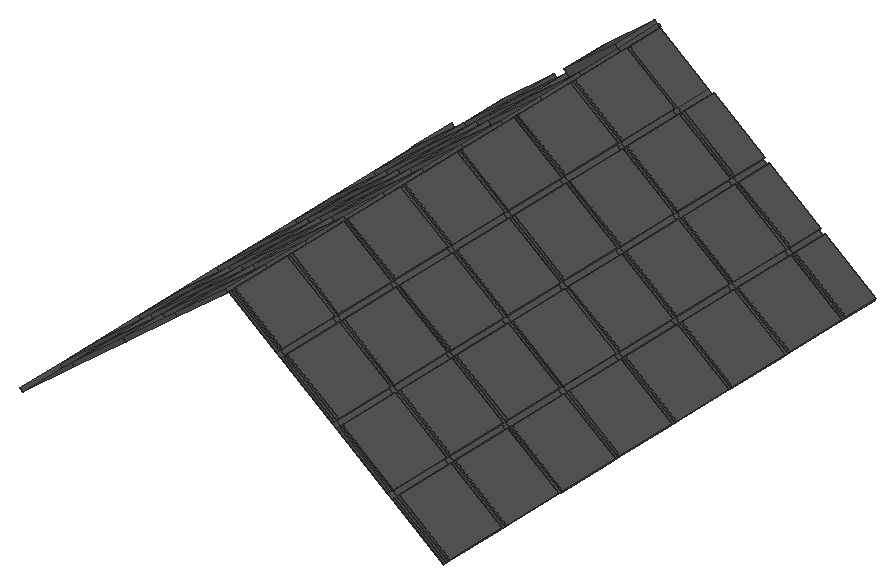
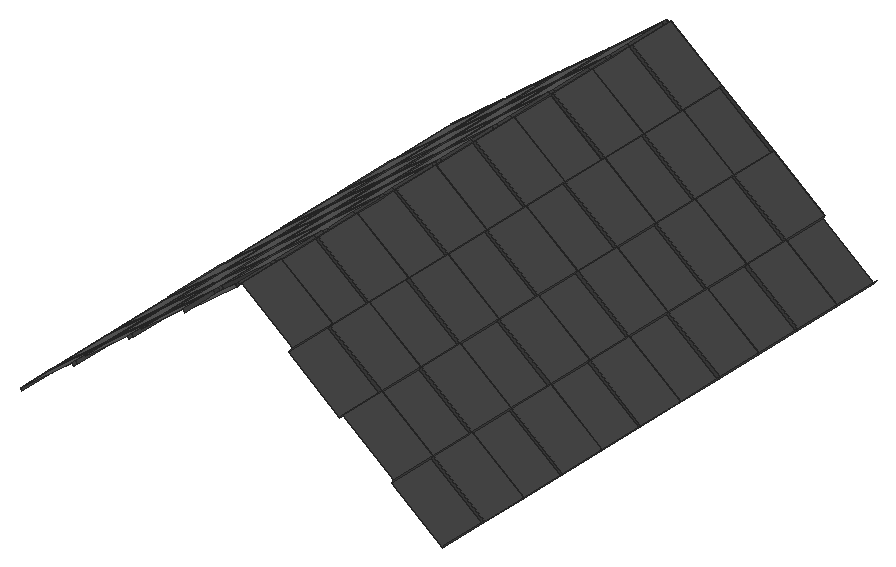
# SketchUp Ruby script. Lengths in inches.
U = 1.inch
M = Sketchup.active_model
def pt(a) = Geom::Point3d.new(a.map { |v| v * U })
def face(e, loops, mat)
  f = e.add_face(loops[0].map { |a| pt(a) })
  loops[1..].each { |l| e.add_face(l.map { |a| pt(a) }).erase! }
  f.material = f.back_material = mat if mat
  f
end
# faces: each face lists its corners as indices into pts; further lists are holes
def faces(e, pts, list, mat = nil) = list.each { |f| face(e, (f[0].is_a?(Array) ? f : [f]).map { |l| l.map { |i| pts[i] } }, mat) }
# xy, xz, yz: faces in a plane at the given z, y or x. An outline is a flat list of corners, or four numbers for a rectangle; further outlines are holes
def ring(l) = l.size == 4 ? [[l[0], l[1]], [l[2], l[1]], [l[2], l[3]], [l[0], l[3]]] : l.each_slice(2).to_a
def flat(e, list, mat, &to3) = list.each { |f| face(e, (f[0].is_a?(Array) ? f : [f]).map { |l| ring(l).map { |u, v| to3.(u, v) } }, mat) }
def xy(e, z, list, mat = nil) = flat(e, list, mat) { |x, y| [x, y, z] }
def xz(e, y, list, mat = nil) = flat(e, list, mat) { |x, z| [x, y, z] }
def yz(e, x, list, mat = nil) = flat(e, list, mat) { |y, z| [x, y, z] }
def lines(e, pts, list) = list.each { |a, b| e.add_line(pt(pts[a]), pt(pts[b])) }
# prism: a flat outline (further loops are holes) pulled along v
def prism(e, loops, v, mat = nil)
  f = face(e, loops, mat); d = Geom::Vector3d.new(v.map { |x| x * U })
  f.pushpull(f.normal.samedirection?(d) ? d.length : -d.length)
end
def box(e, o, s, mat = nil) = prism(e, [[o, [o[0] + s[0], o[1], o[2]], [o[0] + s[0], o[1] + s[1], o[2]], [o[0], o[1] + s[1], o[2]]]], [0, 0, s[2]], mat)
def at(x, y, z, deg = 0) = Geom::Transformation.translation(pt([x, y, z])) * Geom::Transformation.rotation(ORIGIN, Z_AXIS, deg.degrees)
def axes(o, x, y, z) = Geom::Transformation.new([*x, 0, *y, 0, *z, 0, *pt(o).to_a, 1])
def part(name) = M.definitions.add(name)
# library, detail: a bought-in or finely detailed component or shape, given as its bounding box
def library(name, o, s) = part(name).tap { |d| box(d.entities, o, s) }
def detail(e, o, s) = box(e.add_group.entities, o, s)
def put(e, d, t, mat = nil) = e.add_instance(d, t).tap { |i| i.material = mat if mat }
def group(e, t, mat = nil) = e.add_group.tap { |g| g.transformation = t; g.material = mat if mat }.entities
root = M.entities
M.materials.add("[Color M06]").color = [86, 86, 86]
xz(root,343.1875,[[320.63,393.75,339.53,408.54,339.04,409.17,338.73,409.57,319.83,394.78],[339.53,408.54,339.04,409.17,338.73,409.57,357.63,424.36,357.9375,423.97,358.43,423.34],[358.43,423.34,377.33,438.125,376.53,439.15,357.63,424.36,357.9375,423.97]],"[Color M06]")
xz(root,343.375,[[456.38,376.26,437.48,391.05,438.1,391.84,457,377.05],[435.9,392.29,417,407.08,417.62,407.87,436.52,393.07],[415.43,408.3125,396.53,423.1,397.15,423.89,416.05,409.1],[394.95,424.33,377.33,438.125,377.95,438.91,395.57,425.12]],"[Color M06]")
xz(root,345.375,[[456.38,376.26,457,377.05,438.1,391.84,437.48,391.05],[435.9,392.29,436.52,393.07,417.62,407.87,417,407.08],[415.43,408.3125,416.05,409.1,397.15,423.89,396.53,423.1],[394.95,424.33,395.57,425.12,377.95,438.91,377.33,438.125]],"[Color M06]")
xz(root,361.1875,[[301.73,378.96,320.63,393.75,320.14,394.38,319.83,394.78,300.93,379.98,301.24,379.59],[320.63,393.75,320.14,394.38,319.83,394.78,338.73,409.57,339.04,409.17,339.53,408.54],[339.53,408.54,358.43,423.34,357.9375,423.97,357.63,424.36,338.73,409.57,339.04,409.17],[358.43,423.34,357.9375,423.97,357.63,424.36,376.53,439.15,377.33,438.125]],"[Color M06]")
xz(root,369.375,[[456.38,376.26,437.48,391.05,438.1,391.84,457,377.05],[435.9,392.29,417,407.08,417.62,407.87,436.52,393.07],[415.43,408.3125,396.53,423.1,397.15,423.89,416.05,409.1],[394.95,424.33,377.33,438.125,377.95,438.91,395.57,425.12]],"[Color M06]")
xz(root,371.375,[[456.38,376.26,457,377.05,438.1,391.84,437.48,391.05],[435.9,392.29,436.52,393.07,417.62,407.87,417,407.08],[415.43,408.3125,416.05,409.1,397.15,423.89,396.53,423.1],[394.95,424.33,395.57,425.12,377.95,438.91,377.33,438.125]],"[Color M06]")
xz(root,379.1875,[[301.73,378.96,301.24,379.59,300.93,379.98,319.83,394.78,320.14,394.38,320.63,393.75],[320.63,393.75,339.53,408.54,339.04,409.17,338.73,409.57,319.83,394.78,320.14,394.38],[339.53,408.54,339.04,409.17,338.73,409.57,357.63,424.36,357.9375,423.97,358.43,423.34],[358.43,423.34,377.33,438.125,376.53,439.15,357.63,424.36,357.9375,423.97]],"[Color M06]")
xz(root,395.375,[[456.38,376.26,437.48,391.05,438.1,391.84,457,377.05],[435.9,392.29,417,407.08,417.62,407.87,436.52,393.07],[415.43,408.3125,396.53,423.1,397.15,423.89,416.05,409.1],[394.95,424.33,377.33,438.125,377.95,438.91,395.57,425.12]],"[Color M06]")
xz(root,397.1875,[[301.73,378.96,320.63,393.75,320.14,394.38,319.83,394.78,300.93,379.98,301.24,379.59],[320.63,393.75,320.14,394.38,319.83,394.78,338.73,409.57,339.04,409.17,339.53,408.54],[339.53,408.54,358.43,423.34,357.9375,423.97,357.63,424.36,338.73,409.57,339.04,409.17],[358.43,423.34,357.9375,423.97,357.63,424.36,376.53,439.15,377.33,438.125]],"[Color M06]")
xz(root,397.375,[[456.38,376.26,457,377.05,438.1,391.84,437.48,391.05],[435.9,392.29,436.52,393.07,417.62,407.87,417,407.08],[415.43,408.3125,416.05,409.1,397.15,423.89,396.53,423.1],[394.95,424.33,395.57,425.12,377.95,438.91,377.33,438.125]],"[Color M06]")
xz(root,415.1875,[[301.73,378.96,301.24,379.59,300.93,379.98,319.83,394.78,320.63,393.75],[320.63,393.75,339.53,408.54,338.73,409.57,319.83,394.78],[339.53,408.54,338.73,409.57,357.63,424.36,357.9375,423.97,358.43,423.34],[358.43,423.34,377.33,438.125,376.53,439.15,357.63,424.36,357.9375,423.97]],"[Color M06]")
xz(root,421.375,[[456.38,376.26,437.48,391.05,438.1,391.84,457,377.05],[435.9,392.29,417,407.08,417.62,407.87,436.52,393.07],[415.43,408.3125,396.53,423.1,397.15,423.89,416.05,409.1],[394.95,424.33,377.33,438.125,377.95,438.91,395.57,425.12]],"[Color M06]")
xz(root,423.375,[[456.38,376.26,457,377.05,438.1,391.84,437.48,391.05],[435.9,392.29,436.52,393.07,417.62,407.87,417,407.08],[415.43,408.3125,416.05,409.1,397.15,423.89,396.53,423.1],[394.95,424.33,395.57,425.12,377.95,438.91,377.33,438.125]],"[Color M06]")
xz(root,433.1875,[[301.73,378.96,320.63,393.75,319.83,394.78,300.93,379.98,301.24,379.59],[320.63,393.75,319.83,394.78,338.73,409.57,339.53,408.54],[339.53,408.54,358.43,423.34,357.9375,423.97,357.63,424.36,338.73,409.57],[358.43,423.34,357.9375,423.97,357.63,424.36,376.53,439.15,377.33,438.125]],"[Color M06]")
xz(root,447.375,[[456.38,376.26,437.48,391.05,438.1,391.84,457,377.05],[435.9,392.29,417,407.08,417.62,407.87,436.52,393.07],[415.43,408.3125,396.53,423.1,397.15,423.89,416.05,409.1],[394.95,424.33,377.33,438.125,377.95,438.91,395.57,425.12]],"[Color M06]")
xz(root,449.375,[[456.38,376.26,457,377.05,438.1,391.84,437.48,391.05],[435.9,392.29,436.52,393.07,417.62,407.87,417,407.08],[415.43,408.3125,416.05,409.1,397.15,423.89,396.53,423.1],[394.95,424.33,395.57,425.12,377.95,438.91,377.33,438.125]],"[Color M06]")
xz(root,451.1875,[[301.73,378.96,301.24,379.59,300.93,379.98,319.83,394.78,320.14,394.38,320.63,393.75],[320.63,393.75,339.53,408.54,339.04,409.17,338.73,409.57,319.83,394.78,320.14,394.38],[339.53,408.54,339.04,409.17,338.73,409.57,357.63,424.36,358.43,423.34],[358.43,423.34,377.33,438.125,376.53,439.15,357.63,424.36]],"[Color M06]")
xz(root,469.1875,[[301.73,378.96,320.63,393.75,320.14,394.38,319.83,394.78,300.93,379.98,301.24,379.59],[320.63,393.75,320.14,394.38,319.83,394.78,338.73,409.57,339.04,409.17,339.53,408.54],[339.53,408.54,358.43,423.34,357.63,424.36,338.73,409.57,339.04,409.17],[358.43,423.34,357.63,424.36,376.53,439.15,377.33,438.125]],"[Color M06]")
xz(root,473.375,[[456.38,376.26,437.48,391.05,438.1,391.84,457,377.05],[435.9,392.29,417,407.08,417.62,407.87,436.52,393.07],[415.43,408.3125,396.53,423.1,397.15,423.89,416.05,409.1],[394.95,424.33,377.33,438.125,377.95,438.91,395.57,425.12]],"[Color M06]")
xz(root,475.375,[[456.38,376.26,457,377.05,438.1,391.84,437.48,391.05],[435.9,392.29,436.52,393.07,417.62,407.87,417,407.08],[415.43,408.3125,416.05,409.1,397.15,423.89,396.53,423.1],[394.95,424.33,395.57,425.12,377.95,438.91,377.33,438.125]],"[Color M06]")
xz(root,487.1875,[[301.73,378.96,301.24,379.59,300.93,379.98,319.83,394.78,320.14,394.38,320.63,393.75],[320.63,393.75,339.53,408.54,339.04,409.17,338.73,409.57,319.83,394.78,320.14,394.38],[339.53,408.54,339.04,409.17,338.73,409.57,357.63,424.36,358.43,423.34],[358.43,423.34,377.33,438.125,376.53,439.15,357.63,424.36]],"[Color M06]")
xz(root,499.375,[[456.38,376.26,437.48,391.05,438.1,391.84,457,377.05],[435.9,392.29,417,407.08,417.62,407.87,436.52,393.07],[415.43,408.3125,396.53,423.1,397.15,423.89,416.05,409.1],[394.95,424.33,377.33,438.125,377.95,438.91,395.57,425.12]],"[Color M06]")
xz(root,501.375,[[456.38,376.26,457,377.05,438.1,391.84,437.48,391.05],[435.9,392.29,436.52,393.07,417.62,407.87,417,407.08],[415.43,408.3125,416.05,409.1,397.15,423.89,396.53,423.1],[394.95,424.33,395.57,425.12,377.95,438.91,377.33,438.125]],"[Color M06]")
xz(root,505.1875,[[301.73,378.96,320.63,393.75,320.14,394.38,319.83,394.78,300.93,379.98,301.24,379.59],[320.63,393.75,320.14,394.38,319.83,394.78,338.73,409.57,339.04,409.17,339.53,408.54],[339.53,408.54,358.43,423.34,357.63,424.36,338.73,409.57,339.04,409.17],[358.43,423.34,357.63,424.36,376.53,439.15,377.33,438.125]],"[Color M06]")
xz(root,523.1875,[[301.73,378.96,301.24,379.59,300.93,379.98,319.83,394.78,320.14,394.38,320.63,393.75],[320.63,393.75,339.53,408.54,339.04,409.17,338.73,409.57,338.68,409.625,319.78,394.84,319.83,394.78,320.14,394.38],[339.53,408.54,339.04,409.17,338.73,409.57,357.63,424.36,357.9375,423.97,358.43,423.34],[358.43,423.34,377.33,438.125,376.53,439.15,375.68,440.23,356.78,425.44,357.63,424.36,357.9375,423.97]],"[Color M06]")
xz(root,525.375,[[456.38,376.26,437.48,391.05,438.1,391.84,457,377.05],[435.9,392.29,417,407.08,417.62,407.87,436.52,393.07],[415.43,408.3125,396.53,423.1,397.15,423.89,416.05,409.1],[394.95,424.33,377.33,438.125,377.95,438.91,395.57,425.12]],"[Color M06]")
xz(root,527.375,[[456.38,376.26,457,377.05,438.1,391.84,437.48,391.05],[435.9,392.29,436.52,393.07,417.62,407.87,417,407.08],[415.43,408.3125,416.05,409.1,397.15,423.89,396.53,423.1]],"[Color M06]")
xz(root,541.1875,[[377.33,438.125,377.95,438.91,377.09,439.59,376.53,439.15]],"[Color M06]")
p = [[456.38,345.375,376.26],[437.48,345.375,391.05],[437.48,343.375,391.05],[456.38,343.375,376.26],[456.38,369.375,376.26],[457,369.375,377.05],
  [457,345.375,377.05],[456.38,371.375,376.26],[437.48,371.375,391.05],[437.48,369.375,391.05],[456.38,395.375,376.26],[457,395.375,377.05],
  [457,371.375,377.05],[456.38,397.375,376.26],[437.48,397.375,391.05],[437.48,395.375,391.05],[456.38,421.375,376.26],[457,421.375,377.05],
  [457,397.375,377.05],[456.38,423.375,376.26],[437.48,423.375,391.05],[437.48,421.375,391.05],[456.38,447.375,376.26],[457,447.375,377.05],
  [457,423.375,377.05],[456.38,449.375,376.26],[437.48,449.375,391.05],[437.48,447.375,391.05],[456.38,473.375,376.26],[457,473.375,377.05],
  [457,449.375,377.05],[456.38,475.375,376.26],[437.48,475.375,391.05],[437.48,473.375,391.05],[456.38,499.375,376.26],[457,499.375,377.05],
  [457,475.375,377.05],[456.38,501.375,376.26],[437.48,501.375,391.05],[437.48,499.375,391.05],[456.38,525.375,376.26],[457,525.375,377.05],
  [457,501.375,377.05],[456.38,527.375,376.26],[437.48,527.375,391.05],[437.48,525.375,391.05],[456.38,541.1875,376.26],[457,541.1875,377.05],
  [457,527.375,377.05],[438.1,369.375,391.84],[438.1,345.375,391.84],[438.1,395.375,391.84],[438.1,371.375,391.84],[438.1,421.375,391.84],
  [438.1,397.375,391.84],[438.1,447.375,391.84],[438.1,423.375,391.84],[438.1,473.375,391.84],[438.1,449.375,391.84],[438.1,499.375,391.84],
  [438.1,475.375,391.84],[438.1,525.375,391.84],[438.1,501.375,391.84],[438.1,541.1875,391.84],[438.1,527.375,391.84],[301.73,343.1875,378.96],
  [301.73,361.1875,378.96],[301.24,361.1875,379.59],[300.93,361.1875,379.98],[300.93,343.1875,379.98],[320.63,361.1875,393.75],[320.63,343.1875,393.75],
  [301.73,379.1875,378.96],[300.93,379.1875,379.98],[301.24,379.1875,379.59],[301.73,397.1875,378.96],[301.24,397.1875,379.59],[300.93,397.1875,379.98],
  [320.63,397.1875,393.75],[320.63,379.1875,393.75],[301.73,415.1875,378.96],[300.93,415.1875,379.98],[301.24,415.1875,379.59],[301.73,433.1875,378.96],
  [301.24,433.1875,379.59],[300.93,433.1875,379.98],[320.63,433.1875,393.75],[320.63,415.1875,393.75],[301.73,451.1875,378.96],[300.93,451.1875,379.98],
  [301.24,451.1875,379.59],[301.73,469.1875,378.96],[301.24,469.1875,379.59],[300.93,469.1875,379.98],[320.63,469.1875,393.75],[320.63,451.1875,393.75],
  [301.73,487.1875,378.96],[300.93,487.1875,379.98],[301.24,487.1875,379.59],[301.73,505.1875,378.96],[301.24,505.1875,379.59],[300.93,505.1875,379.98],
  [320.63,505.1875,393.75],[320.63,487.1875,393.75],[301.73,523.1875,378.96],[300.93,523.1875,379.98],[301.24,523.1875,379.59],[301.73,541.1875,378.96],
  [300.88,541.1875,380.04],[300.88,523.1875,380.04],[320.63,541.1875,393.75],[320.63,523.1875,393.75],[319.83,379.1875,394.78],[319.83,361.1875,394.78],
  [319.83,415.1875,394.78],[319.83,397.1875,394.78],[319.83,451.1875,394.78],[319.83,433.1875,394.78],[319.83,487.1875,394.78],[319.83,469.1875,394.78],
  [319.83,523.1875,394.78],[319.83,505.1875,394.78],[435.9,343.375,392.29],[435.9,345.375,392.29],[435.9,369.375,392.29],[435.9,371.375,392.29],
  [435.9,395.375,392.29],[435.9,397.375,392.29],[435.9,421.375,392.29],[435.9,423.375,392.29],[435.9,447.375,392.29],[435.9,449.375,392.29],
  [435.9,473.375,392.29],[435.9,475.375,392.29],[435.9,499.375,392.29],[435.9,501.375,392.29],[435.9,525.375,392.29],[435.9,527.375,392.29],
  [437.48,541.1875,391.05],[435.9,541.1875,392.29],[417,345.375,407.08],[417,343.375,407.08],[436.52,369.375,393.07],[436.52,345.375,393.07],
  [417,371.375,407.08],[417,369.375,407.08],[436.52,395.375,393.07],[436.52,371.375,393.07],[417,397.375,407.08],[417,395.375,407.08],
  [436.52,421.375,393.07],[436.52,397.375,393.07],[417,423.375,407.08],[417,421.375,407.08],[436.52,447.375,393.07],[436.52,423.375,393.07],
  [417,449.375,407.08],[417,447.375,407.08],[436.52,473.375,393.07],[436.52,449.375,393.07],[417,475.375,407.08],[417,473.375,407.08],
  [436.52,499.375,393.07],[436.52,475.375,393.07],[417,501.375,407.08],[417,499.375,407.08],[436.52,525.375,393.07],[436.52,501.375,393.07],
  [417,527.375,407.08],[417,525.375,407.08],[436.52,541.1875,393.07],[436.52,527.375,393.07],[417.62,369.375,407.87],[417.62,345.375,407.87],
  [417.62,395.375,407.87],[417.62,371.375,407.87],[417.62,421.375,407.87],[417.62,397.375,407.87],[417.62,447.375,407.87],[417.62,423.375,407.87],
  [417.62,473.375,407.87],[417.62,449.375,407.87],[417.62,499.375,407.87],[417.62,475.375,407.87],[417.62,525.375,407.87],[417.62,501.375,407.87],
  [417.62,541.1875,407.87],[417.62,527.375,407.87],[319.83,343.1875,394.78],[320.14,361.1875,394.38],[320.14,379.1875,394.38],[339.53,379.1875,408.54],
  [339.53,361.1875,408.54],[320.14,397.1875,394.38],[339.53,415.1875,408.54],[339.53,397.1875,408.54],[320.14,451.1875,394.38],[339.53,451.1875,408.54],
  [339.53,433.1875,408.54],[320.14,469.1875,394.38],[320.14,487.1875,394.38],[339.53,487.1875,408.54],[339.53,469.1875,408.54],[320.14,505.1875,394.38],
  [320.14,523.1875,394.38],[339.53,523.1875,408.54],[339.53,505.1875,408.54],[319.78,523.1875,394.84],[319.78,541.1875,394.84],[338.73,361.1875,409.57],
  [338.73,343.1875,409.57],[338.73,397.1875,409.57],[338.73,379.1875,409.57],[338.73,433.1875,409.57],[338.73,415.1875,409.57],[338.73,469.1875,409.57],
  [338.73,451.1875,409.57],[338.73,505.1875,409.57],[338.73,487.1875,409.57],[338.68,541.1875,409.625],[338.68,523.1875,409.625],[415.43,345.375,408.3125],
  [415.43,343.375,408.3125],[415.43,369.375,408.3125],[415.43,371.375,408.3125],[415.43,395.375,408.3125],[415.43,397.375,408.3125],[415.43,421.375,408.3125],
  [415.43,423.375,408.3125],[415.43,447.375,408.3125],[415.43,449.375,408.3125],[415.43,473.375,408.3125],[415.43,475.375,408.3125],[415.43,499.375,408.3125],
  [415.43,501.375,408.3125],[415.43,525.375,408.3125],[415.43,527.375,408.3125],[417,541.1875,407.08],[415.43,541.1875,408.3125],[396.53,345.375,423.1],
  [396.53,343.375,423.1],[416.05,369.375,409.1],[416.05,345.375,409.1],[396.53,371.375,423.1],[396.53,369.375,423.1],[416.05,395.375,409.1],
  [416.05,371.375,409.1],[396.53,397.375,423.1],[396.53,395.375,423.1],[416.05,421.375,409.1],[416.05,397.375,409.1],[396.53,423.375,423.1],
  [396.53,421.375,423.1],[416.05,447.375,409.1],[416.05,423.375,409.1],[396.53,449.375,423.1],[396.53,447.375,423.1],[416.05,473.375,409.1],
  [416.05,449.375,409.1],[396.53,475.375,423.1],[396.53,473.375,423.1],[416.05,499.375,409.1],[416.05,475.375,409.1],[396.53,501.375,423.1],
  [396.53,499.375,423.1],[416.05,525.375,409.1],[416.05,501.375,409.1],[396.53,527.375,423.1],[396.53,525.375,423.1],[416.05,541.1875,409.1],
  [416.05,527.375,409.1],[339.53,343.1875,408.54],[339.04,361.1875,409.17],[339.04,343.1875,409.17],[358.43,361.1875,423.34],[358.43,343.1875,423.34],
  [339.04,379.1875,409.17],[339.04,397.1875,409.17],[358.43,397.1875,423.34],[358.43,379.1875,423.34],[358.43,433.1875,423.34],[358.43,415.1875,423.34],
  [339.04,451.1875,409.17],[339.04,469.1875,409.17],[358.43,469.1875,423.34],[358.43,451.1875,423.34],[339.04,487.1875,409.17],[339.04,505.1875,409.17],
  [358.43,505.1875,423.34],[358.43,487.1875,423.34],[338.73,523.1875,409.57],[339.04,523.1875,409.17],[339.53,541.1875,408.54],[358.43,541.1875,423.34],
  [358.43,523.1875,423.34],[397.15,369.375,423.89],[397.15,345.375,423.89],[397.15,395.375,423.89],[397.15,371.375,423.89],[397.15,421.375,423.89],
  [397.15,397.375,423.89],[397.15,447.375,423.89],[397.15,423.375,423.89],[397.15,473.375,423.89],[397.15,449.375,423.89],[397.15,499.375,423.89],
  [397.15,475.375,423.89],[397.15,525.375,423.89],[397.15,501.375,423.89],[397.15,541.1875,423.89],[397.15,527.375,423.89],[357.63,379.1875,424.36],
  [357.63,361.1875,424.36],[357.63,415.1875,424.36],[357.63,397.1875,424.36],[357.63,451.1875,424.36],[357.63,433.1875,424.36],[357.63,487.1875,424.36],
  [357.63,469.1875,424.36],[357.63,523.1875,424.36],[357.63,505.1875,424.36],[394.95,345.375,424.33],[394.95,343.375,424.33],[394.95,369.375,424.33],
  [394.95,371.375,424.33],[394.95,395.375,424.33],[394.95,397.375,424.33],[394.95,421.375,424.33],[394.95,423.375,424.33],[394.95,447.375,424.33],
  [394.95,449.375,424.33],[394.95,473.375,424.33],[394.95,475.375,424.33],[394.95,499.375,424.33],[394.95,501.375,424.33],[394.95,525.375,424.33],
  [394.95,527.375,424.33],[396.53,541.1875,423.1],[394.95,541.1875,424.33],[357.9375,343.1875,423.97],[357.63,343.1875,424.36],[357.9375,361.1875,423.97],
  [357.9375,379.1875,423.97],[377.33,379.1875,438.125],[377.33,361.1875,438.125],[377.33,369.375,438.125],[377.33,371.375,438.125],[357.9375,397.1875,423.97],
  [377.33,395.375,438.125],[377.33,397.1875,438.125],[357.9375,415.1875,423.97],[377.33,415.1875,438.125],[377.33,397.375,438.125],[357.9375,433.1875,423.97],
  [377.33,451.1875,438.125],[377.33,433.1875,438.125],[377.33,447.375,438.125],[377.33,449.375,438.125],[377.33,487.1875,438.125],[377.33,469.1875,438.125],
  [377.33,473.375,438.125],[377.33,475.375,438.125],[357.9375,523.1875,423.97],[377.33,523.1875,438.125],[377.33,505.1875,438.125],[356.78,523.1875,425.44],
  [356.78,541.1875,425.44],[377.33,343.375,438.125],[377.33,345.375,438.125],[395.57,369.375,425.12],[395.57,345.375,425.12],[395.57,395.375,425.12],
  [395.57,371.375,425.12],[395.57,421.375,425.12],[395.57,397.375,425.12],[377.33,421.375,438.125],[377.33,423.375,438.125],[395.57,447.375,425.12],
  [395.57,423.375,425.12],[395.57,473.375,425.12],[395.57,449.375,425.12],[395.57,499.375,425.12],[395.57,475.375,425.12],[377.33,499.375,438.125],
  [377.33,501.375,438.125],[395.57,525.375,425.12],[395.57,501.375,425.12],[377.33,525.375,438.125],[377.33,527.375,438.125],[377.33,541.1875,438.125],
  [376.53,361.1875,439.15],[376.53,343.1875,439.15],[376.53,397.1875,439.15],[376.53,379.1875,439.15],[376.53,433.1875,439.15],[376.53,415.1875,439.15],
  [376.53,469.1875,439.15],[376.53,451.1875,439.15],[376.53,505.1875,439.15],[376.53,487.1875,439.15],[377.95,345.375,438.91],[377.95,369.375,438.91],
  [377.95,361.1875,438.91],[377.95,371.375,438.91],[377.95,395.375,438.91],[377.95,379.1875,438.91],[377.95,397.375,438.91],[377.95,421.375,438.91],
  [377.95,415.1875,438.91],[377.95,423.375,438.91],[377.95,447.375,438.91],[377.95,433.1875,438.91],[377.95,449.375,438.91],[377.95,473.375,438.91],
  [377.95,469.1875,438.91],[377.95,451.1875,438.91],[377.95,475.375,438.91],[377.95,499.375,438.91],[377.95,487.1875,438.91],[377.95,501.375,438.91],
  [377.95,525.375,438.91],[377.95,523.1875,438.91],[377.95,505.1875,438.91],[375.68,541.1875,440.23],[375.68,523.1875,440.23],[377.33,343.1875,438.125],
  [377.95,343.1875,438.91],[377.95,343.375,438.91],[376.53,523.1875,439.15],[376.53,541.1875,439.15],[377.95,541.1875,438.91]]
faces(root,p,[[0,1,2,3],[0,4,5,6],[7,8,9,4],[7,10,11,12],[13,14,15,10],[13,16,17,18],[19,20,21,16],[19,22,23,24],
  [25,26,27,22],[25,28,29,30],[31,32,33,28],[31,34,35,36],[37,38,39,34],[37,40,41,42],[43,44,45,40],[43,46,47,48],
  [5,49,50,6],[11,51,52,12],[17,53,54,18],[23,55,56,24],[29,57,58,30],[35,59,60,36],[41,61,62,42],[47,63,64,48],
  [65,66,67,68,69],[70,66,65,71],[72,66,67,68,73,74],[72,75,76,77,73,74],[78,75,72,79],[80,75,76,77,81,82],[80,83,84,85,81,82],[86,83,80,87],
  [88,83,84,85,89,90],[88,91,92,93,89,90],[94,91,88,95],[96,91,92,93,97,98],[96,99,100,101,97,98],[102,99,96,103],[104,99,100,101,105,106],[104,107,108,109,105,106],
  [110,107,104,111],[112,73,68,113],[114,81,77,115],[116,89,85,117],[118,97,93,119],[120,105,101,121],[122,2,1,123],[123,1,9,124],
  [9,1,50,49],[124,9,8,125],[125,8,15,126],[15,8,52,51],[126,15,14,127],[21,128,127,14],[21,14,54,53],[128,21,20,129],
  [129,20,27,130],[27,20,56,55],[26,131,130,27],[33,132,131,26],[33,26,58,57],[32,133,132,33],[39,134,133,32],[39,32,60,59],
  [38,135,134,39],[45,136,135,38],[45,38,62,61],[44,137,136,45],[138,139,137,44],[138,44,64,63],[123,140,141,122],[123,124,142,143],
  [125,144,145,124],[125,126,146,147],[127,148,149,126],[127,128,150,151],[129,152,153,128],[129,130,154,155],[131,156,157,130],[131,132,158,159],
  [133,160,161,132],[133,134,162,163],[135,164,165,134],[135,136,166,167],[137,168,169,136],[137,139,170,171],[142,172,173,143],[146,174,175,147],
  [150,176,177,151],[154,178,179,155],[158,180,181,159],[162,182,183,163],[166,184,185,167],[170,186,187,171],[70,71,188,113,189],[70,79,190,112,113,189],
  [191,79,70,192],[78,79,190,112,115,193],[78,87,114,115,193],[194,87,78,195],[86,87,114,117],[86,95,196,116,117],[197,95,86,198],[94,95,196,116,119,199],
  [94,103,200,118,119,199],[201,103,94,202],[102,103,200,118,121,203],[102,111,204,120,121,203],[205,111,102,206],[110,111,204,120,207,208],[209,113,188,210],[211,115,112,212],
  [213,117,114,214],[215,119,116,216],[217,121,118,218],[219,208,207,220],[140,221,222,141],[145,223,221,140],[145,140,173,172],[144,224,223,145],
  [149,225,224,144],[149,144,175,174],[225,149,148,226],[226,148,153,227],[153,148,177,176],[227,153,152,228],[228,152,157,229],[157,152,179,178],
  [229,157,156,230],[230,156,161,231],[161,156,181,180],[231,161,160,232],[165,233,232,160],[165,160,183,182],[233,165,164,234],[234,164,169,235],
  [169,164,185,184],[168,236,235,169],[236,168,237,238],[237,168,187,186],[221,239,240,222],[221,223,241,242],[224,243,244,223],[224,225,245,246],
  [226,247,248,225],[226,227,249,250],[228,251,252,227],[228,229,253,254],[230,255,256,229],[230,231,257,258],[232,259,260,231],[232,233,261,262],
  [234,263,264,233],[234,235,265,266],[236,267,268,235],[236,238,269,270],[271,192,272,209,210,273],[274,192,271,275],[191,192,272,209,212,276],[191,195,277,211,212,276],
  [278,195,191,279],[194,195,277,211,214],[194,198,213,214],[280,198,194,281],[197,198,213,216,282],[197,202,283,215,216,282],[284,202,197,285],[201,202,283,215,218,286],
  [201,206,287,217,218,286],[288,206,201,289],[205,206,287,217,290,291],[205,292,219,220,290,291],[293,292,205,294],[241,295,296,242],[245,297,298,246],[249,299,300,250],
  [253,301,302,254],[257,303,304,258],[261,305,306,262],[265,307,308,266],[269,309,310,270],[311,212,209,312],[313,214,211,314],[315,216,213,316],
  [317,218,215,318],[319,290,217,320],[239,321,322,240],[244,323,321,239],[244,239,296,295],[243,324,323,244],[248,325,324,243],[248,243,298,297],
  [325,248,247,326],[252,327,326,247],[252,247,300,299],[251,328,327,252],[256,329,328,251],[256,251,302,301],[329,256,255,330],[260,331,330,255],
  [260,255,304,303],[259,332,331,260],[332,259,264,333],[264,259,306,305],[263,334,333,264],[334,263,268,335],[268,263,308,307],[335,268,267,336],
  [336,267,337,338],[337,267,310,309],[274,275,339,340,312,341],[274,279,342,311,312,341],[343,279,274,344,345,346],[278,279,342,311,314,347],[348,349,278,279,343],[278,281,350,313,314,347],
  [351,281,278,349,352],[280,281,350,313,316,353],[280,285,315,316,353],[354,285,280,355,356,357],[284,285,315,318],[284,289,317,318],[358,289,284,359,360,361],[288,289,317,320],
  [288,294,362,319,320],[363,294,288,364],[293,294,362,319,365,366],[367,322,321,368],[321,323,369,370],[345,323,324,346],[324,325,371,372],[348,325,326,352,349],
  [326,327,373,374],[375,327,328,376],[328,329,377,378],[356,329,330,357],[330,331,379,380],[360,331,332,361],[332,333,381,382],[383,333,334,384],
  [334,335,385,386],[387,335,336,388],[388,336,338,389],[390,312,340,391],[392,314,311,393],[394,316,313,395],[396,318,315,397],[398,320,317,399],
  [400,370,369,401,402],[403,372,371,404,405],[406,374,373,407,408],[409,378,377,410,411],[412,380,379,413,414,415],[416,382,381,417,418],[419,386,385,420,421,422],[423,366,365,424],
  [425,367,368,344,390,391],[367,425,426,427],[368,367,427,400],[344,368,400,402],[393,390,344,345,346,343],[345,344,402,401],[346,345,401,403],[343,346,403,405],
  [343,348,349,392,393],[348,343,405,404],[349,348,404,406,352],[395,392,349,352,351],[351,352,406,408],[351,375,376,355,394,395],[375,351,408,407],[376,375,407,409],
  [355,376,409,411],[397,394,355,356,357,354],[356,355,411,410],[357,356,410,412],[354,357,412,415],[354,359,396,397],[359,354,415,414],[399,396,359,360,361,358],
  [360,359,414,413],[361,360,413,416],[358,361,416,418],[358,383,384,364,398,399],[383,358,418,417],[384,383,417,419],[364,384,419,422],[428,398,364,363],
  [363,364,422,421],[389,429,428,363,387,388],[387,363,421,420],[388,387,420,430,389],[424,428,429,423]],"[Color M06]")
